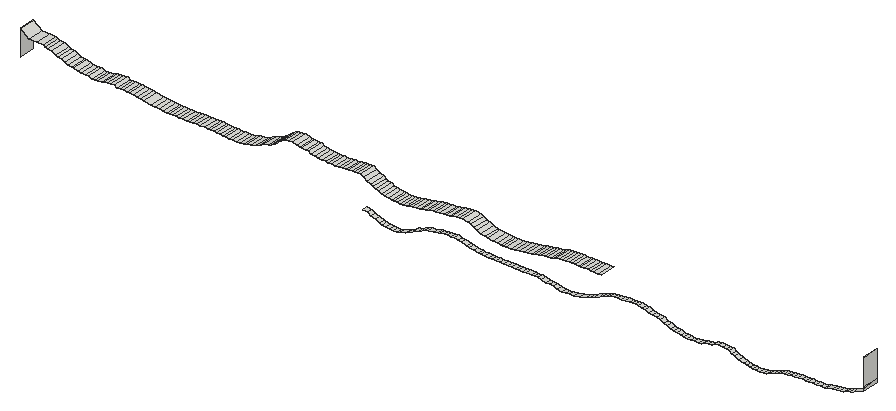
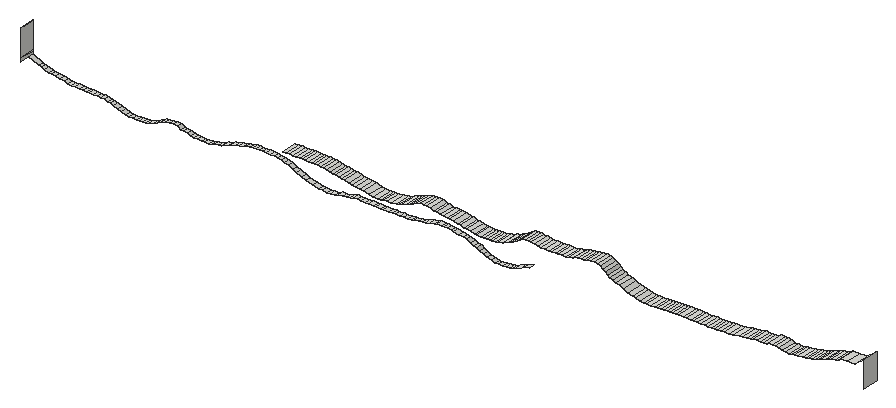
# SketchUp Ruby script. Lengths in inches.
U = 1.inch
M = Sketchup.active_model
def pt(a) = Geom::Point3d.new(a.map { |v| v * U })
def face(e, loops, mat)
  f = e.add_face(loops[0].map { |a| pt(a) })
  loops[1..].each { |l| e.add_face(l.map { |a| pt(a) }).erase! }
  f.material = f.back_material = mat if mat
  f
end
# faces: each face lists its corners as indices into pts; further lists are holes
def faces(e, pts, list, mat = nil) = list.each { |f| face(e, (f[0].is_a?(Array) ? f : [f]).map { |l| l.map { |i| pts[i] } }, mat) }
# xy, xz, yz: faces in a plane at the given z, y or x. An outline is a flat list of corners, or four numbers for a rectangle; further outlines are holes
def ring(l) = l.size == 4 ? [[l[0], l[1]], [l[2], l[1]], [l[2], l[3]], [l[0], l[3]]] : l.each_slice(2).to_a
def flat(e, list, mat, &to3) = list.each { |f| face(e, (f[0].is_a?(Array) ? f : [f]).map { |l| ring(l).map { |u, v| to3.(u, v) } }, mat) }
def xy(e, z, list, mat = nil) = flat(e, list, mat) { |x, y| [x, y, z] }
def xz(e, y, list, mat = nil) = flat(e, list, mat) { |x, z| [x, y, z] }
def yz(e, x, list, mat = nil) = flat(e, list, mat) { |y, z| [x, y, z] }
def lines(e, pts, list) = list.each { |a, b| e.add_line(pt(pts[a]), pt(pts[b])) }
# prism: a flat outline (further loops are holes) pulled along v
def prism(e, loops, v, mat = nil)
  f = face(e, loops, mat); d = Geom::Vector3d.new(v.map { |x| x * U })
  f.pushpull(f.normal.samedirection?(d) ? d.length : -d.length)
end
def box(e, o, s, mat = nil) = prism(e, [[o, [o[0] + s[0], o[1], o[2]], [o[0] + s[0], o[1] + s[1], o[2]], [o[0], o[1] + s[1], o[2]]]], [0, 0, s[2]], mat)
def at(x, y, z, deg = 0) = Geom::Transformation.translation(pt([x, y, z])) * Geom::Transformation.rotation(ORIGIN, Z_AXIS, deg.degrees)
def axes(o, x, y, z) = Geom::Transformation.new([*x, 0, *y, 0, *z, 0, *pt(o).to_a, 1])
def part(name) = M.definitions.add(name)
# library, detail: a bought-in or finely detailed component or shape, given as its bounding box
def library(name, o, s) = part(name).tap { |d| box(d.entities, o, s) }
def detail(e, o, s) = box(e.add_group.entities, o, s)
def put(e, d, t, mat = nil) = e.add_instance(d, t).tap { |i| i.material = mat if mat }
def group(e, t, mat = nil) = e.add_group.tap { |g| g.transformation = t; g.material = mat if mat }.entities
root = M.entities
xy(root,238.18,[[2133.53,565.74,2134.21,566.68]])
xy(root,238.62,[[2100.06,565.74,2100.83,566.68],[2100.83,565.74,2101.46,566.68],[2101.46,565.74,2102.22,566.68],[2102.22,565.74,2102.84,566.68],[2102.84,565.74,2103.69,566.68],
  [2103.69,565.74,2104.33,566.68],[2104.33,565.74,2104.95,566.68]])
xy(root,238.625,[[2098.64,565.74,2099.5,566.68]])
xy(root,238.89,[[2154.45,565.74,2155.13,566.68]])
xy(root,238.9,[[2155.89,565.74,2156.51,566.68],[2156.51,565.74,2157.28,566.68]])
xy(root,240.43,[[2122.73,565.74,2123.3,566.68]])
xy(root,241.68,[[2040.78,565.74,2041.37,568.68]])
xy(root,241.75,[[2043.13,565.74,2044,568.68],[2044,565.74,2044.62,568.68],[2044.62,565.74,2045.13,568.68]])
xy(root,243.05,[[2115.79,565.74,2116.47,568.68]])
xy(root,243.07,[[2113.9375,565.74,2114.52,568.68]])
xy(root,243.09,[[2110.625,565.74,2111.15,568.68],[2111.15,565.74,2111.67,568.68],[2111.67,565.74,2112.33,568.68],[2112.33,565.74,2112.78,568.68]])
yz(root,2010.34,[[565.74,241.52,568.68,246.2]])
yz(root,2164.35,[[565.74,240.89,565.74,241.29,568.68,241.52,568.68,240.89],[565.74,241.29,568.68,241.52,565.74,241.52],[565.74,241.52,565.74,246.27,566.4375,246.36,568.68,246.43,568.68,241.52],[565.74,246.27,565.74,246.43,568.68,246.43,566.4375,246.36]])
p = [[2077.14,565.74,237.11],[2077.14,566.68,237.11],[2077.9,566.68,237.04],[2077.9,565.74,237.04],[2078.59,566.68,237.01],[2078.59,565.74,237.01],
  [2079.2,566.68,236.98],[2079.2,565.74,236.98],[2079.88,566.68,237.22],[2079.88,565.74,237.22],[2076.45,565.74,237.2],[2076.45,566.68,237.2],
  [2075.92,565.74,237.33],[2075.92,566.68,237.33],[2080.73,566.68,237.43],[2080.73,565.74,237.43],[2075.25,565.74,237.68],[2075.25,566.68,237.68],
  [2081.35,566.68,237.74],[2081.35,565.74,237.74],[2144.18,565.74,237.45],[2144.18,566.68,237.45],[2144.75,566.68,237.42],[2144.75,565.74,237.42],
  [2145.48,566.68,237.4],[2145.48,565.74,237.4],[2146.16,566.68,237.47],[2146.16,565.74,237.47],[2142.99,565.74,237.59],[2142.99,566.68,237.59],
  [2143.59,566.68,237.51],[2143.59,565.74,237.51],[2146.76,566.68,237.5625],[2146.76,565.74,237.5625],[2142.45,565.74,237.71],[2142.45,566.68,237.71],
  [2147.45,566.68,237.84],[2147.45,565.74,237.84],[2074.3125,565.74,237.96],[2074.3125,566.68,237.96],[2082.05,566.68,238.02],[2082.05,565.74,238.02],
  [2109.19,565.74,237.79],[2109.19,566.68,237.79],[2109.9,566.68,237.74],[2109.9,565.74,237.74],[2110.77,566.68,237.87],[2110.77,565.74,237.87],
  [2141.62,565.74,238],[2141.62,566.68,238],[2108.42,565.74,237.86],[2108.42,566.68,237.86],[2148.13,566.68,238.08],[2148.13,565.74,238.08],
  [2107.79,565.74,238.15],[2107.79,566.68,238.15],[2111.42,566.68,237.88],[2111.42,565.74,237.88],[2112.54,566.68,238.14],[2112.54,565.74,238.14],
  [2073.75,565.74,238.28],[2073.75,566.68,238.28],[2082.49,566.68,238.375],[2082.49,565.74,238.375],[2140.91,565.74,238.33],[2140.91,566.68,238.33],
  [2107.02,565.74,238.19],[2107.02,566.68,238.19],[2113.76,566.68,238.46],[2113.76,565.74,238.46],[2131.51,565.74,238.19],[2131.51,566.68,238.19],
  [2132.33,566.68,238.15],[2132.33,565.74,238.15],[2132.86,566.68,238.11],[2132.86,565.74,238.11],[2133.53,566.68,238.18],[2133.53,565.74,238.18],
  [2148.82,566.68,238.33],[2148.82,565.74,238.33],[2106.4,565.74,238.25],[2106.4,566.68,238.25],[2130.9375,565.74,238.26],[2130.9375,566.68,238.26],
  [2134.21,565.74,238.18],[2134.21,566.68,238.18],[2134.89,566.68,238.27],[2134.89,565.74,238.27],[2072.97,565.74,238.43],[2072.97,566.68,238.43],
  [2105.64,565.74,238.45],[2105.64,566.68,238.45],[2130.37,565.74,238.48],[2130.37,566.68,238.48],[2135.41,566.68,238.55],[2135.41,565.74,238.55],
  [2140.36,565.74,238.57],[2140.36,566.68,238.57],[2149.35,566.68,238.51],[2149.35,565.74,238.51],[2083.05,566.68,238.51],[2083.05,565.74,238.51],
  [2083.6875,566.68,238.76],[2083.6875,565.74,238.76],[2104.95,565.74,238.62],[2104.95,566.68,238.62],[2114.51,566.68,238.72],[2114.51,565.74,238.72],
  [2129.71,565.74,238.56],[2129.71,566.68,238.56],[2136.07,566.68,238.61],[2136.07,565.74,238.61],[2149.92,566.68,238.6],[2149.92,565.74,238.6],
  [2095.88,565.74,238.66],[2095.88,566.68,238.66],[2096.55,566.68,238.65],[2096.55,565.74,238.65],[2097.33,566.68,238.64],[2097.33,565.74,238.64],
  [2097.95,566.68,238.63],[2097.95,565.74,238.63],[2098.64,566.68,238.625],[2098.64,565.74,238.625],[2099.5,565.74,238.625],[2099.5,566.68,238.625],
  [2100.06,566.68,238.62],[2100.06,565.74,238.62],[2129.14,565.74,238.67],[2129.14,566.68,238.67],[2136.66,566.68,238.66],[2136.66,565.74,238.66],
  [2139.86,565.74,238.86],[2139.86,566.68,238.86],[2150.58,566.68,238.74],[2150.58,565.74,238.74],[2094.04,565.74,238.78],[2094.04,566.68,238.78],
  [2094.52,566.68,238.73],[2094.52,565.74,238.73],[2095.19,566.68,238.6875],[2095.19,565.74,238.6875],[2115.39,566.68,239.08],[2115.39,565.74,239.08],
  [2128.62,565.74,239.01],[2128.62,566.68,239.01],[2137.23,566.68,239.04],[2137.23,565.74,239.04],[2151.16,566.68,238.8],[2151.16,565.74,238.8],
  [2084.33,566.68,239.12],[2084.33,565.74,239.12],[2093.16,565.74,238.93],[2093.16,566.68,238.93],[2151.73,566.68,238.83],[2151.73,565.74,238.83],
  [2152.47,566.68,238.86],[2152.47,565.74,238.86],[2092.39,565.74,239.07],[2092.39,566.68,239.07],[2139.34,565.74,238.96],[2139.34,566.68,238.96],
  [2153.23,566.68,238.875],[2153.23,565.74,238.875],[2153.77,566.68,238.88],[2153.77,565.74,238.88],[2154.45,566.68,238.89],[2154.45,565.74,238.89],
  [2155.13,565.74,238.89],[2155.13,566.68,238.89],[2155.89,566.68,238.9],[2155.89,565.74,238.9],[2157.28,565.74,238.9],[2157.28,566.68,238.9],
  [2157.91,566.68,239.15],[2157.91,565.74,239.15],[2127.9375,565.74,239.18],[2127.9375,566.68,239.18],[2137.97,566.68,239.125],[2137.97,565.74,239.125],
  [2138.65,566.68,239.02],[2138.65,565.74,239.02],[2084.91,566.68,239.22],[2084.91,565.74,239.22],[2091.84,565.74,239.16],[2091.84,566.68,239.16],
  [2116.18,566.68,239.375],[2116.18,565.74,239.375],[2085.91,566.68,239.31],[2085.91,565.74,239.31],[2090.99,565.74,239.44],[2090.99,566.68,239.44],
  [2127.3125,565.74,239.5],[2127.3125,566.68,239.5],[2158.68,566.68,239.28],[2158.68,565.74,239.28],[2086.72,566.68,239.54],[2086.72,565.74,239.54],
  [2159.48,566.68,239.42],[2159.48,565.74,239.42],[2090.32,565.74,239.56],[2090.32,566.68,239.56],[2116.92,566.68,239.75],[2116.92,565.74,239.75],
  [2160.2,566.68,239.49],[2160.2,565.74,239.49],[2087.21,566.68,239.6],[2087.21,565.74,239.6],[2126.55,565.74,239.65],[2126.55,566.68,239.65],
  [2160.75,566.68,239.53],[2160.75,565.74,239.53],[2161.4375,566.68,239.81],[2161.4375,565.74,239.81],[2087.83,566.68,239.65],[2087.83,565.74,239.65],
  [2088.42,566.68,239.69],[2088.42,565.74,239.69],[2089.71,565.74,239.72],[2089.71,566.68,239.72],[2088.98,566.68,239.7],[2088.98,565.74,239.7],
  [2117.57,566.68,239.97],[2117.57,565.74,239.97],[2125.9375,565.74,239.8],[2125.9375,566.68,239.8],[2125.18,565.74,239.96],[2125.18,566.68,239.96],
  [2161.96,566.68,239.96],[2161.96,565.74,239.96],[2118.19,566.68,240.17],[2118.19,565.74,240.17],[2124.53,565.74,240.23],[2124.53,566.68,240.23],
  [2162.52,566.68,240.1],[2162.52,565.74,240.1],[2164.35,566.68,240.89],[2164.35,565.74,240.89],[2118.87,566.68,240.27],[2118.87,565.74,240.27],
  [2123.95,565.74,240.27],[2123.95,566.68,240.27],[2119.55,566.68,240.33],[2119.55,565.74,240.33],[2120.24,566.68,240.37],[2120.24,565.74,240.37],
  [2123.3,565.74,240.43],[2123.3,566.68,240.43],[2120.93,566.68,240.4],[2120.93,565.74,240.4],[2121.625,566.68,240.41],[2121.625,565.74,240.41],
  [2122.15,566.68,240.42],[2122.15,565.74,240.42],[2122.73,566.68,240.43],[2122.73,565.74,240.43],[2046.76,568.68,241.57],[2047.3,568.68,241.53],
  [2047.3,565.74,241.53],[2046.76,565.74,241.57],[2047.92,568.68,241.51],[2047.92,565.74,241.51],[2048.47,568.68,241.49],[2048.47,565.74,241.49],
  [2049.17,568.68,241.48],[2049.17,565.74,241.48],[2049.83,568.68,241.47],[2049.83,565.74,241.47],[2050.4,568.68,241.46],[2050.4,565.74,241.46],
  [2051.11,568.68,241.6],[2051.11,565.74,241.6],[2097.48,568.68,241.56],[2098.08,568.68,241.51],[2098.08,565.74,241.51],[2097.48,565.74,241.56],
  [2098.53,568.68,241.48],[2098.53,565.74,241.48],[2099.05,568.68,241.46],[2099.05,565.74,241.46],[2099.92,568.68,241.51],[2099.92,565.74,241.51],
  [2100.64,568.68,241.59],[2100.64,565.74,241.59],[2046.15,568.68,241.66],[2046.15,565.74,241.66],[2051.84,568.68,241.85],[2051.84,565.74,241.85],
  [2095.66,568.68,241.78],[2096.71,568.68,241.63],[2096.71,565.74,241.63],[2095.66,565.74,241.78],[2101.58,568.68,241.82],[2101.58,565.74,241.82],
  [2037.12,568.68,241.75],[2037.57,568.68,241.74],[2037.57,565.74,241.74],[2037.12,565.74,241.75],[2038.12,568.68,241.72],[2038.12,565.74,241.72],
  [2038.75,568.68,241.71],[2038.75,565.74,241.71],[2039.38,568.68,241.7],[2039.38,565.74,241.7],[2040.11,568.68,241.69],[2040.11,565.74,241.69],
  [2040.78,568.68,241.68],[2040.78,565.74,241.68],[2041.37,568.68,241.68],[2041.86,568.68,241.67],[2041.86,565.74,241.67],[2041.37,565.74,241.68],
  [2042.5625,568.68,241.74],[2042.5625,565.74,241.74],[2043.13,568.68,241.75],[2043.13,565.74,241.75],[2045.13,568.68,241.75],[2045.62,568.68,241.67],
  [2045.62,565.74,241.67],[2045.13,565.74,241.75],[2034.93,568.68,241.89],[2035.75,568.68,241.83],[2035.75,565.74,241.83],[2034.93,565.74,241.89],
  [2036.35,568.68,241.78],[2036.35,565.74,241.78],[2052.51,568.68,241.91],[2052.51,565.74,241.91],[2078.14,568.68,241.89],[2078.6,568.68,241.85],
  [2078.6,565.74,241.85],[2078.14,565.74,241.89],[2079.12,568.68,241.8125],[2079.12,565.74,241.8125],[2079.63,568.68,241.79],[2079.63,565.74,241.79],
  [2080.21,568.68,241.78],[2080.21,565.74,241.78],[2080.88,568.68,241.91],[2080.88,565.74,241.91],[2095.17,568.68,241.89],[2095.17,565.74,241.89],
  [2102.36,568.68,241.87],[2102.36,565.74,241.87],[2034.16,568.68,241.96],[2034.16,565.74,241.96],[2053.41,568.68,242.1],[2053.41,565.74,242.1],
  [2077.58,568.68,241.96],[2077.58,565.74,241.96],[2081.35,568.68,241.93],[2081.35,565.74,241.93],[2082.02,568.68,242.09],[2082.02,565.74,242.09],
  [2094.53,568.68,242.14],[2094.53,565.74,242.14],[2103.125,568.68,241.98],[2103.125,565.74,241.98],[2032.99,568.68,242.24],[2032.99,565.74,242.24],
  [2076.9,568.68,242.11],[2076.9,565.74,242.11],[2103.74,568.68,242.02],[2103.74,565.74,242.02],[2104.39,568.68,242.19],[2104.39,565.74,242.19],
  [2054.18,568.68,242.46],[2054.18,565.74,242.46],[2076.3,568.68,242.21],[2076.3,565.74,242.21],[2082.79,568.68,242.2],[2082.79,565.74,242.2],
  [2093.77,568.68,242.39],[2093.77,565.74,242.39],[2032.32,568.68,242.34],[2032.32,565.74,242.34],[2075.79,568.68,242.51],[2075.79,565.74,242.51],
  [2083.29,568.68,242.24],[2083.29,565.74,242.24],[2083.9,568.68,242.42],[2083.9,565.74,242.42],[2105.09,568.68,242.38],[2105.09,565.74,242.38],
  [2031.66,568.68,242.38],[2031.66,565.74,242.38],[2031,568.68,242.48],[2031,565.74,242.48],[2084.45,568.68,242.47],[2084.45,565.74,242.47],
  [2093.15,568.68,242.65],[2093.15,565.74,242.65],[2105.58,568.68,242.4375],[2105.58,565.74,242.4375],[2106.1,568.68,242.48],[2106.1,565.74,242.48],
  [2022.82,568.68,242.68],[2023.49,568.68,242.51],[2023.49,565.74,242.51],[2022.82,565.74,242.68],[2024.01,568.68,242.46],[2024.01,565.74,242.46],
  [2024.55,568.68,242.58],[2024.55,565.74,242.58],[2030.36,568.68,242.57],[2030.36,565.74,242.57],[2054.88,568.68,242.78],[2054.88,565.74,242.78],
  [2075.2,568.68,242.68],[2075.2,565.74,242.68],[2085.2,568.68,242.71],[2085.2,565.74,242.71],[2106.76,568.68,242.58],[2106.76,565.74,242.58],
  [2025.18,568.68,242.57],[2025.18,565.74,242.57],[2025.81,568.68,242.81],[2025.81,565.74,242.81],[2027.58,568.68,242.92],[2028.01,568.68,242.625],
  [2028.01,565.74,242.625],[2027.58,565.74,242.92],[2028.62,568.68,242.65],[2028.62,565.74,242.65],[2029.17,568.68,242.62],[2029.17,565.74,242.62],
  [2029.8,568.68,242.58],[2029.8,565.74,242.58],[2092.6,568.68,242.9375],[2092.6,565.74,242.9375],[2107.29,568.68,242.61],[2107.29,565.74,242.61],
  [2107.875,568.68,242.77],[2107.875,565.74,242.77],[2021.47,568.68,242.78],[2022.28,568.68,242.73],[2022.28,565.74,242.73],[2021.47,565.74,242.78],
  [2074.7,568.68,242.875],[2074.7,565.74,242.875],[2085.84,568.68,242.78],[2085.84,565.74,242.78],[2020.17,568.68,243.06],[2020.89,568.68,242.85],
  [2020.89,565.74,242.85],[2020.17,565.74,243.06],[2026.38,568.68,242.86],[2026.38,565.74,242.86],[2055.65,568.68,242.97],[2055.65,565.74,242.97],
  [2086.32,568.68,242.82],[2086.32,565.74,242.82],[2087.01,568.68,242.85],[2087.01,565.74,242.85],[2108.33,568.68,242.95],[2108.33,565.74,242.95],
  [2026.94,568.68,242.89],[2026.94,565.74,242.89],[2074.31,568.68,243.09],[2074.31,565.74,243.09],[2087.71,568.68,242.87],[2087.71,565.74,242.87],
  [2088.26,568.68,243.02],[2088.26,565.74,243.02],[2092.03,568.68,243.14],[2092.03,565.74,243.14],[2056.18,568.68,243.23],[2056.18,565.74,243.23],
  [2088.88,568.68,243.05],[2088.88,565.74,243.05],[2108.89,568.68,243.01],[2108.89,565.74,243.01],[2109.4,568.68,243.05],[2109.4,565.74,243.05],
  [2109.97,568.68,243.08],[2109.97,565.74,243.08],[2019.1,568.68,243.3],[2019.6875,568.68,243.14],[2019.6875,565.74,243.14],[2019.1,565.74,243.3],
  [2073.7,568.68,243.43],[2073.7,565.74,243.43],[2089.43,568.68,243.29],[2089.43,565.74,243.29],[2091.26,568.68,243.42],[2091.26,565.74,243.42],
  [2110.625,568.68,243.09],[2110.625,565.74,243.09],[2112.78,568.68,243.09],[2113.35,568.68,243.08],[2113.35,565.74,243.08],[2112.78,565.74,243.09],
  [2113.9375,568.68,243.07],[2113.9375,565.74,243.07],[2114.52,568.68,243.07],[2115.18,568.68,243.0625],[2115.18,565.74,243.0625],[2114.52,565.74,243.07],
  [2115.79,568.68,243.05],[2115.79,565.74,243.05],[2056.58,568.68,243.48],[2056.58,565.74,243.48],[2018.46,568.68,243.48],[2018.46,565.74,243.48],
  [2090.11,568.68,243.35],[2090.11,565.74,243.35],[2073.16,568.68,243.8],[2073.16,565.74,243.8],[2090.66,568.68,243.39],[2090.66,565.74,243.39],
  [2017.94,568.68,243.79],[2017.94,565.74,243.79],[2057.1,568.68,243.72],[2057.1,565.74,243.72],[2057.4375,568.68,244.12],[2057.4375,565.74,244.12],
  [2017.28,568.68,243.95],[2017.28,565.74,243.95],[2072.56,568.68,244.18],[2072.56,565.74,244.18],[2016.76,568.68,244.11],[2016.76,565.74,244.11],
  [2065.38,568.68,243.99],[2066.1,568.68,243.95],[2066.1,565.74,243.95],[2065.38,565.74,243.99],[2066.6,568.68,243.93],[2066.6,565.74,243.93],
  [2067.29,568.68,243.91],[2067.29,565.74,243.91],[2067.86,568.68,243.89],[2067.86,565.74,243.89],[2068.56,568.68,243.88],[2068.56,565.74,243.88],
  [2069.21,568.68,243.94],[2069.21,565.74,243.94],[2069.85,568.68,243.95],[2069.85,565.74,243.95],[2070.41,568.68,244.1],[2070.41,565.74,244.1],
  [2064.2,568.68,244.11],[2064.76,568.68,244.04],[2064.76,565.74,244.04],[2064.2,565.74,244.11],[2016.09,568.68,244.41],[2016.09,565.74,244.41],
  [2057.91,568.68,244.39],[2057.91,565.74,244.39],[2063.45,568.68,244.25],[2063.45,565.74,244.25],[2071.04,568.68,244.13],[2071.04,565.74,244.13],
  [2071.52,568.68,244.15],[2071.52,565.74,244.15],[2072.04,568.68,244.17],[2072.04,565.74,244.17],[2062.99,568.68,244.51],[2062.99,565.74,244.51],
  [2015.33,568.68,244.54],[2015.33,565.74,244.54],[2058.39,568.68,244.73],[2058.39,565.74,244.73],[2014.77,568.68,244.61],[2014.77,565.74,244.61],
  [2061.84,568.68,244.67],[2062.45,568.68,244.55],[2062.45,565.74,244.55],[2061.84,565.74,244.67],[2014.55,568.68,244.92],[2014.55,565.74,244.92],
  [2058.875,568.68,244.87],[2058.875,565.74,244.87],[2060.79,568.68,244.81],[2061.36,568.68,244.7],[2061.36,565.74,244.7],[2060.79,565.74,244.81],
  [2060.14,568.68,245.01],[2060.14,565.74,245.01],[2011.91,568.68,244.96],[2013.3,568.68,244.9375],[2013.3,565.74,244.9375],[2011.91,565.74,244.96],
  [2059.46,568.68,244.95],[2059.46,565.74,244.95],[2010.34,568.68,246.2],[2010.34,565.74,246.2]]
faces(root,p,[[0,1,2,3],[3,2,4,5],[5,4,6,7],[7,6,8,9],[10,11,1,0],[12,13,11,10],[9,8,14,15],[16,17,13,12],
  [15,14,18,19],[20,21,22,23],[23,22,24,25],[25,24,26,27],[28,29,30,31],[31,30,21,20],[27,26,32,33],[34,35,29,28],
  [33,32,36,37],[38,39,17,16],[19,18,40,41],[42,43,44,45],[45,44,46,47],[48,49,35,34],[50,51,43,42],[37,36,52,53],
  [54,55,51,50],[47,46,56,57],[57,56,58,59],[60,61,39,38],[41,40,62,63],[64,65,49,48],[66,67,55,54],[59,58,68,69],
  [70,71,72,73],[73,72,74,75],[75,74,76,77],[53,52,78,79],[80,81,67,66],[82,83,71,70],[84,85,86,87],[88,89,61,60],
  [90,91,81,80],[92,93,83,82],[87,86,94,95],[96,97,65,64],[79,78,98,99],[63,62,100,101],[101,100,102,103],[104,105,91,90],
  [69,68,106,107],[108,109,93,92],[95,94,110,111],[99,98,112,113],[114,115,116,117],[117,116,118,119],[119,118,120,121],[121,120,122,123],
  [124,125,126,127],[128,129,109,108],[111,110,130,131],[132,133,97,96],[113,112,134,135],[136,137,138,139],[139,138,140,141],[141,140,115,114],
  [107,106,142,143],[144,145,129,128],[131,130,146,147],[135,134,148,149],[103,102,150,151],[152,153,137,136],[149,148,154,155],[155,154,156,157],
  [158,159,153,152],[160,161,133,132],[157,156,162,163],[163,162,164,165],[165,164,166,167],[168,169,170,171],[172,173,174,175],[176,177,145,144],
  [147,146,178,179],[179,178,180,181],[181,180,161,160],[151,150,182,183],[184,185,159,158],[143,142,186,187],[183,182,188,189],[190,191,185,184],
  [192,193,177,176],[175,174,194,195],[189,188,196,197],[195,194,198,199],[200,201,191,190],[187,186,202,203],[199,198,204,205],[197,196,206,207],
  [208,209,193,192],[205,204,210,211],[211,210,212,213],[207,206,214,215],[215,214,216,217],[218,219,201,200],[217,216,220,221],[221,220,219,218],
  [203,202,222,223],[224,225,209,208],[226,227,225,224],[213,212,228,229],[223,222,230,231],[232,233,227,226],[229,228,234,235],[235,234,236,237],
  [231,230,238,239],[240,241,233,232],[239,238,242,243],[243,242,244,245],[246,247,241,240],[245,244,248,249],[249,248,250,251],[251,250,252,253],
  [253,252,254,255],[256,257,258,259],[257,260,261,258],[260,262,263,261],[262,264,265,263],[264,266,267,265],[266,268,269,267],[268,270,271,269],
  [272,273,274,275],[273,276,277,274],[276,278,279,277],[278,280,281,279],[280,282,283,281],[284,256,259,285],[270,286,287,271],[288,289,290,291],
  [289,272,275,290],[282,292,293,283],[294,295,296,297],[295,298,299,296],[298,300,301,299],[300,302,303,301],[302,304,305,303],[304,306,307,305],
  [308,309,310,311],[309,312,313,310],[312,314,315,313],[316,317,318,319],[317,284,285,318],[320,321,322,323],[321,324,325,322],[324,294,297,325],
  [286,326,327,287],[328,329,330,331],[329,332,333,330],[332,334,335,333],[334,336,337,335],[336,338,339,337],[340,288,291,341],[292,342,343,293],
  [344,320,323,345],[326,346,347,327],[348,328,331,349],[338,350,351,339],[350,352,353,351],[354,340,341,355],[342,356,357,343],[358,344,345,359],
  [360,348,349,361],[356,362,363,357],[362,364,365,363],[346,366,367,347],[368,360,361,369],[352,370,371,353],[372,354,355,373],[374,358,359,375],
  [376,368,369,377],[370,378,379,371],[378,380,381,379],[364,382,383,365],[384,374,375,385],[386,384,385,387],[380,388,389,381],[390,372,373,391],
  [382,392,393,383],[392,394,395,393],[396,397,398,399],[397,400,401,398],[400,402,403,401],[404,386,387,405],[366,406,407,367],[408,376,377,409],
  [388,410,411,389],[394,412,413,395],[402,414,415,403],[414,416,417,415],[418,419,420,421],[419,422,423,420],[422,424,425,423],[424,426,427,425],
  [426,404,405,427],[428,390,391,429],[412,430,431,413],[430,432,433,431],[434,435,436,437],[435,396,399,436],[438,408,409,439],[410,440,441,411],
  [442,443,444,445],[443,434,437,444],[416,446,447,417],[406,448,449,407],[440,450,451,441],[450,452,453,451],[432,454,455,433],[446,456,457,447],
  [456,418,421,457],[458,438,439,459],[452,460,461,453],[460,462,463,461],[464,428,429,465],[448,466,467,449],[462,468,469,463],[454,470,471,455],
  [470,472,473,471],[472,474,475,473],[476,477,478,479],[477,442,445,478],[480,458,459,481],[468,482,483,469],[484,464,465,485],[474,486,487,475],
  [488,489,490,491],[489,492,493,490],[494,495,496,497],[495,498,499,496],[466,500,501,467],[502,476,479,503],[482,504,505,483],[506,480,481,507],
  [504,508,509,505],[508,484,485,509],[510,502,503,511],[500,512,513,501],[512,514,515,513],[516,510,511,517],[518,506,507,519],[520,516,517,521],
  [522,523,524,525],[523,526,527,524],[526,528,529,527],[528,530,531,529],[530,532,533,531],[532,534,535,533],[534,536,537,535],[536,538,539,537],
  [540,541,542,543],[541,522,525,542],[544,520,521,545],[514,546,547,515],[548,540,543,549],[538,550,551,539],[550,552,553,551],[552,554,555,553],
  [554,518,519,555],[556,548,549,557],[558,544,545,559],[546,560,561,547],[562,558,559,563],[564,565,566,567],[565,556,557,566],[568,562,563,569],
  [560,570,571,561],[572,573,574,575],[573,564,567,574],[576,572,575,577],[578,579,580,581],[579,568,569,580],[570,582,583,571],[582,576,577,583],
  [584,578,581,585]])
